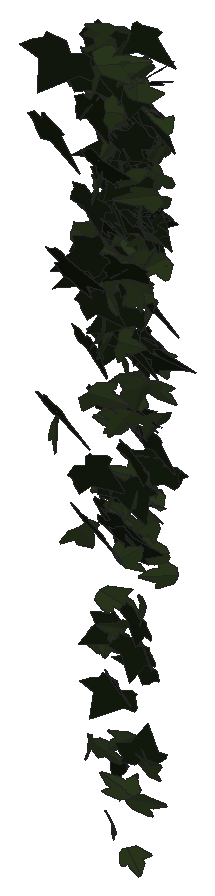
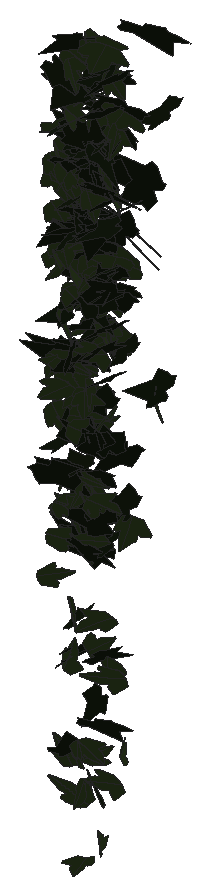
# SketchUp Ruby script. Lengths in millimetres.
U = 1.mm
M = Sketchup.active_model
def pt(a) = Geom::Point3d.new(a.map { |v| v * U })
def face(e, loops, mat)
  f = e.add_face(loops[0].map { |a| pt(a) })
  loops[1..].each { |l| e.add_face(l.map { |a| pt(a) }).erase! }
  f.material = f.back_material = mat if mat
  f
end
# faces: each face lists its corners as indices into pts; further lists are holes
def faces(e, pts, list, mat = nil) = list.each { |f| face(e, (f[0].is_a?(Array) ? f : [f]).map { |l| l.map { |i| pts[i] } }, mat) }
# xy, xz, yz: faces in a plane at the given z, y or x. An outline is a flat list of corners, or four numbers for a rectangle; further outlines are holes
def ring(l) = l.size == 4 ? [[l[0], l[1]], [l[2], l[1]], [l[2], l[3]], [l[0], l[3]]] : l.each_slice(2).to_a
def flat(e, list, mat, &to3) = list.each { |f| face(e, (f[0].is_a?(Array) ? f : [f]).map { |l| ring(l).map { |u, v| to3.(u, v) } }, mat) }
def xy(e, z, list, mat = nil) = flat(e, list, mat) { |x, y| [x, y, z] }
def xz(e, y, list, mat = nil) = flat(e, list, mat) { |x, z| [x, y, z] }
def yz(e, x, list, mat = nil) = flat(e, list, mat) { |y, z| [x, y, z] }
def lines(e, pts, list) = list.each { |a, b| e.add_line(pt(pts[a]), pt(pts[b])) }
# prism: a flat outline (further loops are holes) pulled along v
def prism(e, loops, v, mat = nil)
  f = face(e, loops, mat); d = Geom::Vector3d.new(v.map { |x| x * U })
  f.pushpull(f.normal.samedirection?(d) ? d.length : -d.length)
end
def box(e, o, s, mat = nil) = prism(e, [[o, [o[0] + s[0], o[1], o[2]], [o[0] + s[0], o[1] + s[1], o[2]], [o[0], o[1] + s[1], o[2]]]], [0, 0, s[2]], mat)
def at(x, y, z, deg = 0) = Geom::Transformation.translation(pt([x, y, z])) * Geom::Transformation.rotation(ORIGIN, Z_AXIS, deg.degrees)
def axes(o, x, y, z) = Geom::Transformation.new([*x, 0, *y, 0, *z, 0, *pt(o).to_a, 1])
def part(name) = M.definitions.add(name)
# library, detail: a bought-in or finely detailed component or shape, given as its bounding box
def library(name, o, s) = part(name).tap { |d| box(d.entities, o, s) }
def detail(e, o, s) = box(e.add_group.entities, o, s)
def put(e, d, t, mat = nil) = e.add_instance(d, t).tap { |i| i.material = mat if mat }
def group(e, t, mat = nil) = e.add_group.tap { |g| g.transformation = t; g.material = mat if mat }.entities
root = M.entities
M.materials.add("efeu1").color = [18, 25, 13]
M.materials.add("efeu2").color = [43, 57, 29]
c1 = part("ivyleaf_10")
p = [[0,12.8,-0.8],[-1.5,51.3,-10.9],[-4.9,51,-11.6],[-13.6,26.5,-7.3],[-13.2,15.9,-4.6],[-21.1,19.3,-7.2],
  [-29.5,16.3,-8.3],[-29.2,8.3,-6.2],[-19.7,-9.8,0.5],[-7.6,-13,4],[1,-12.2,5.8],[-0.4,51.1,-11.1],
  [-1.5,51.1,-10.9],[1,-12.4,5.9],[16.9,-12.4,3.5],[35.1,9.1,-5.1],[35,12.9,-6.1],[20.5,16.4,-4.9],
  [15.8,15,-3.8],[15.3,27.6,-7.1],[12.8,31.3,-7.8]]
faces(c1.entities,p,[[0,1,2,3,4,5,6,7,8,9,10],[11,12,0,13,14,15,16,17,18,19,20]],"efeu2")
c2 = part("ivyleaf_9")
p = [[39.1,54.8,31.7],[34.5,51.8,30.2],[-5.3,25.2,17.3],[-17.9,28.3,20.9],[-21.6,21.7,17],[-20.2,4.3,5.3],
  [-22.9,-0.3,2.5],[-17.1,-4,-0.6],[-2,-2.1,-1.2],[-0.7,-15.4,-10.1],[16.6,-22.3,-16.7],[21.1,-15.1,-12.5],
  [32.7,-10.7,-11],[46.1,-1.8,-6.6],[30.8,11.2,3.8]]
faces(c2.entities,p,[[0,1,2,3,4,5,6,7,8,9,10,11,12,13,14]],"efeu1")
put(root,c1,axes([1822.5,943,1481.1],[-0.28005,-0.67314,-0.56509],[0.19497,0.55591,-0.68889],[1.6613,-0.17872,-0.01441]))
put(root,c2,axes([1797.8,841.9,1483.6],[0.91084,-0.90282,-0.01651],[-0.00863,0.01629,-1.02182],[1.71851,0.47859,0.00362]))
put(root,c1,axes([1800.7,982.2,265.7],[-0.64136,0.11442,-0.62069],[1.10096,-0.2254,-0.35563],[-0.48039,-0.66934,0.01365]))
put(root,c2,axes([1805.6,976.5,1322.7],[1.1743,-0.35369,-0.29662],[-0.21622,0.36357,-0.66985],[0.8515,0.58009,0.23897]))
put(root,c2,axes([1832.1,990.5,375.3],[-1.32874,-0.41465,-0.00161],[0.01139,-0.00692,-0.81196],[0.78909,-0.69813,0.00901]))
put(root,c1,axes([1799.8,976.6,463.8],[-0.35998,-0.04208,-0.70449],[1.31314,0.14236,-0.19375],[0.28248,-0.71542,0.00288]))
put(root,c2,axes([1809.5,962.5,1601.2],[0.50907,-0.59476,-0.53681],[-0.20226,0.53459,-0.64527],[1.51135,0.27188,0.09446]))
put(root,c2,axes([1848.5,985.5,1385.8],[-1.38044,0.01635,0.30216],[-0.57495,-0.08465,-0.72058],[0.03342,-0.78117,0.08441]))
put(root,c2,axes([1815.6,968.9,1205],[-0.84219,-0.53442,-0.4027],[0.57762,0.26999,-0.6918],[1.13503,-0.53394,0.05325]))
put(root,c2,axes([1821.2,991.6,1028.3],[-0.43094,-0.70313,0.32913],[-0.17988,-0.31533,-0.73866],[1.46656,-0.24529,0.00611]))
put(root,c2,axes([1808.6,971,1131.2],[0.66553,-0.51406,-0.57933],[-0.15789,0.60713,-0.5888],[1.46559,0.29884,0.19964]))
put(root,c2,axes([1824.8,969.7,1180.9],[0.65454,-0.28914,-0.66596],[-0.91808,0.45971,-0.44871],[1.03266,0.59198,0.02318]))
put(root,c1,axes([1807.4,948.9,1522.4],[1.59505,0.02697,0.36476],[0.69401,0.0092,-0.83852],[-0.05405,0.91398,-0.00232]))
put(root,c1,axes([1830.5,953.2,1584.5],[-0.20352,-0.75394,0.33237],[-0.00832,-0.33464,-0.76049],[1.56813,-0.09963,0.0391]))
put(root,c2,axes([1841.8,974.9,1454.1],[-0.45993,0.76746,0.00714],[-0.00313,0.00697,-0.80461],[-1.46068,-0.24166,-0.00052]))
put(root,c2,axes([1798.8,853.1,959.1],[1.0734,-0.75753,0.18315],[0.21065,-0.14594,-0.94443],[1.46825,0.57475,0.0016]))
put(root,c2,axes([1838.6,980.8,493.7],[-0.77235,-0.44111,0.56041],[-0.71215,-0.41723,-0.59936],[1.15552,-0.55197,0.00519]))
put(root,c2,axes([1807.2,970.2,1194.7],[-0.1034,-0.1559,-0.79226],[0.67159,0.70962,-0.16383],[1.38222,-0.35645,0.02034]))
put(root,c1,axes([1818.5,954.9,1244.4],[1.19737,0.42133,0.11867],[0.16739,0.08188,-0.75695],[-0.81609,0.63497,0.01886]))
put(root,c2,axes([1810.4,979.1,718.9],[0.86688,-0.63563,-0.11104],[-0.12018,0.09135,-0.78198],[1.22216,0.45984,0.00186]))
put(root,c2,axes([1810.2,983.5,901.5],[-0.25854,-0.26803,0.76169],[0.66502,-0.71584,-0.18958],[1.38544,0.29359,0.23314]))
put(root,c1,axes([1818.7,935.2,294.5],[0.06632,-0.01536,0.72305],[0.69663,-0.62395,-0.03089],[1.18711,0.36701,-0.02227]))
put(root,c1,axes([1797.2,939.3,1232.4],[0.25186,-0.01742,0.84861],[1.60609,0.09486,-0.12965],[-0.17334,0.85361,0.03173]))
put(root,c1,axes([1813.9,851.1,925.9],[0.48896,-0.3956,0.84112],[0.97579,-0.66758,-0.47059],[1.47557,0.57256,0.03248]))
put(root,c1,axes([1821.9,972.2,1396],[0.53535,-0.52689,0.55434],[0.53485,-0.47812,-0.59704],[1.35372,0.39727,0.01667]))
put(root,c1,axes([1823,965.1,486.7],[1.22149,-0.19109,0.18532],[0.33707,-0.05457,-0.66965],[0.37822,0.66579,-0.0017]))
put(root,c1,axes([1831,897.6,713.3],[-0.62595,-0.76075,-0.42534],[0.39043,0.37428,-0.82805],[1.6122,-0.38601,0.03539]))
put(root,c2,axes([1840.2,984.2,1072.1],[-0.59749,-0.46681,0.63515],[-0.67582,-0.52662,-0.56255],[1.33933,-0.47397,-0.00051]))
put(root,c2,axes([1807.6,943.5,1536.2],[-0.03607,-0.43085,-0.7109],[1.00024,0.54472,-0.34415],[1.22575,-0.45718,0.25991]))
put(root,c1,axes([1844,978,783.3],[-0.4931,-0.3786,0.71299],[-0.26314,-0.71693,-0.43094],[1.5137,-0.24796,0.15735]))
put(root,c2,axes([1809.1,972.2,1180.6],[0.9158,-0.58167,0.28923],[0.36311,-0.21752,-0.75486],[1.18181,0.51757,0.0078]))
put(root,c2,axes([1825.3,971.6,1359.1],[0.29639,-0.74503,-0.27025],[-0.12894,0.2619,-0.76104],[1.50283,0.16941,-0.01199]))
put(root,c2,axes([1847.8,842.5,1626.5],[-1.75835,-0.45387,-0.15194],[0.26022,0.06627,-1.02935],[0.87296,-0.93395,0.0008]))
put(root,c1,axes([1850.8,975.5,503.2],[-0.38759,-0.1579,-0.65503],[-0.69128,-0.55063,0.24566],[-1.08008,0.40908,0.07783]))
put(root,c2,axes([1859.6,963.4,240.5],[-0.55829,0.20895,-0.70547],[-1.16698,0.35034,0.35873],[0.77395,0.67897,0.032]))
put(root,c1,axes([1836.3,973.6,1124.6],[0.01605,-0.18199,0.7631],[0.40521,-0.73397,-0.1774],[1.43703,0.209,0.0415]))
put(root,c2,axes([1820.6,923.5,1052.3],[0.45536,-0.74582,0.36603],[0.15434,-0.35812,-0.78272],[1.57363,0.25094,-0.02915]))
put(root,c1,axes([1842,963.1,922.1],[-0.25016,0.57468,0.54752],[0.1665,-0.5411,0.58895],[1.50145,0.15575,0.02591]))
put(root,c2,axes([1830.2,979.5,1225],[-0.22156,-0.7799,0.28254],[0.08433,-0.29074,-0.7843],[1.57645,-0.09406,0.08166]))
put(root,c2,axes([1828.8,924.6,1321.6],[-0.02349,-0.81617,0.10867],[0.0394,-0.10895,-0.81596],[1.56655,-0.0095,0.02215]))
put(root,c1,axes([1828.9,977.7,131.6],[-0.35685,0.08828,0.63772],[0.83068,-0.47084,0.19351],[0.90071,0.46921,0.07419]))
put(root,c1,axes([1860.2,933.7,1488.3],[-1.3551,0.11709,0.42797],[-0.81604,0.02654,-0.72061],[-0.21718,-0.83031,0.03732]))
put(root,c1,axes([1847.5,954.4,1412],[0.21003,-0.84178,-0.35734],[-0.06931,0.3556,-0.84893],[1.73907,0.11584,0.00932]))
put(root,c2,axes([1832.4,974.7,1530.9],[-0.19851,-0.80782,-0.10846],[0.03186,0.1072,-0.81452],[1.55092,-0.1056,0.00285]))
put(root,c2,axes([1831.1,946.9,1213.4],[0.94597,-0.38709,-0.5058],[-0.45391,0.4818,-0.60309],[1.124,0.52034,0.18214]))
put(root,c2,axes([1824.1,932,1489.5],[-0.53964,-0.16781,-0.80142],[1.55793,-0.03867,-0.28152],[0.0357,-0.84922,0.17118]))
put(root,c1,axes([1839.2,935.7,1353.4],[0.56258,-0.62662,0.51847],[0.42502,-0.46791,-0.69284],[1.48839,0.37047,0.00187]))
put(root,c2,axes([1837.2,968.8,1440.7],[-0.30047,-0.49117,0.63866],[0.01681,-0.65182,-0.49911],[1.53329,-0.08911,0.13063]))
put(root,c2,axes([1820.7,930.9,1281.7],[0.3083,-0.37225,0.7742],[0.69931,-0.68211,-0.40485],[1.47782,0.40044,0.03006]))
put(root,c2,axes([1858.6,974.8,1162.7],[-0.58438,0.64426,-0.3801],[0.3307,-0.3382,-0.71362],[-1.38471,-0.35266,-0.01002]))
put(root,c1,axes([1853.3,980.5,1363.8],[-0.25887,-0.80427,-0.03819],[-0.00137,0.03885,-0.81566],[1.53242,-0.13583,-0.00718]))
put(root,c1,axes([1831.7,967.6,560.8],[0.56824,0.42412,0.62452],[0.58902,0.54379,-0.51725],[-1.31047,0.42832,0.03831]))
put(root,c2,axes([1846,962.8,407.6],[1.14893,-0.26922,-0.47629],[-0.83014,0.19133,-0.66099],[0.62859,0.74477,-0.00236]))
put(root,c2,axes([1824.5,982.3,893.2],[-0.00837,0.01,0.7808],[1.31996,-0.35873,0.0085],[0.68288,0.69353,-0.00686]))
put(root,c1,axes([1855.5,959.5,1498.5],[-0.26483,-0.74986,0.33585],[0.07633,-0.34643,-0.75686],[1.56188,-0.11022,0.09394]))
put(root,c1,axes([1829.6,977.8,715.6],[0.57678,0.07748,0.6264],[1.12171,0.21391,-0.31161],[-0.42985,0.66217,0.02737]))
put(root,c1,axes([1835.1,980.9,1072.2],[-0.85041,0.0973,-0.60337],[1.05014,-0.25716,-0.4501],[-0.50015,-0.70539,0.08087]))
put(root,c1,axes([1870.6,938.8,1630.9],[-1.16692,-0.45216,0.3727],[-0.50315,-0.26795,-0.76],[0.99525,-0.66562,0.05277]))
put(root,c2,axes([1841.7,910.3,1148.3],[0.52178,-0.5404,-0.6401],[-0.27287,0.6333,-0.59607],[1.57081,0.28952,0.10908]))
put(root,c1,axes([1861.3,912.1,1087.4],[0.15621,-0.72855,-0.48451],[-0.0897,0.48225,-0.73314],[1.66279,0.09446,0.00597]))
put(root,c1,axes([1854.2,943.5,1625.9],[-1.2911,-0.4395,-0.24822],[0.4042,0.12868,-0.80828],[0.87146,-0.71082,0.00715]))
put(root,c2,axes([1851.9,973.9,1428.4],[-0.46239,0.17122,-0.76702],[1.07645,-0.51932,-0.29508],[-1.03848,-0.61454,0.03566]))
put(root,c2,axes([1857.1,986.5,699.8],[-1.28707,-0.11085,-0.41353],[0.77393,0.07549,-0.68525],[0.25485,-0.78908,-0.00747]))
put(root,c2,axes([1846.3,941.8,1575.7],[-0.48594,-0.75949,-0.34593],[0.29742,0.31185,-0.80001],[1.56024,-0.29599,0.04476]))
put(root,c1,axes([1861.8,972.6,998.7],[0.6302,-0.44636,-0.5607],[-0.13184,0.59483,-0.51444],[1.35758,0.26497,0.21032]))
put(root,c2,axes([1828.6,955,1235.7],[0.26393,-0.13524,-0.79554],[1.19089,0.52773,0.01937],[0.96977,-0.61125,0.19273]))
put(root,c1,axes([1852.4,963.7,1211.1],[-0.41267,-0.52961,-0.55132],[0.5706,0.46825,-0.56772],[1.33841,-0.36292,0.07205]))
put(root,c2,axes([1850.6,984.9,1165.4],[-0.16514,-0.62892,0.45455],[-0.07873,-0.45299,-0.63465],[1.47476,-0.09461,0.01702]))
put(root,c2,axes([1828,972.4,748.1],[0.84176,-0.04822,0.63431],[1.19663,-0.08427,-0.44482],[0.184,0.76867,-0.00898]))
put(root,c1,axes([1873,972.9,309.3],[-0.6641,-0.40693,0.41414],[-0.49373,-0.32299,-0.53595],[0.98857,-0.43468,0.01053]))
put(root,c1,axes([1859.5,942.9,1426.2],[0.89336,-0.69261,0.04582],[0.04127,-0.04066,-0.83667],[1.32041,0.46988,-0.00485]))
put(root,c1,axes([1864.6,952.8,1433.1],[-0.27859,-0.67822,0.52747],[0.04806,-0.53823,-0.68505],[1.6345,-0.09977,0.11005]))
put(root,c1,axes([1856.5,971.8,908.1],[0.10651,-0.34727,0.61371],[0.39166,-0.5808,-0.34741],[1.28362,0.20603,0.05508]))
put(root,c1,axes([1857.6,913.9,1573.6],[0.19868,-0.73708,0.41387],[0.37639,-0.38414,-0.73402],[1.56417,0.18606,0.12406]))
put(root,c1,axes([1865.6,971.4,1232],[-0.32409,-0.73889,-0.09967],[0.01445,0.10052,-0.75811],[1.41892,-0.16979,-0.01505]))
put(root,c2,axes([1847.2,969.5,1297.5],[0.15955,-0.67692,-0.36171],[0.09908,0.36804,-0.6767],[1.45734,0.04909,0.0856]))
put(root,c2,axes([1852.4,886,842.6],[0.24473,-0.32835,-0.91099],[-0.41175,0.88602,-0.34989],[1.79639,0.24781,0.04391]))
put(root,c2,axes([1864.7,952.5,1297.8],[1.33185,0.05372,-0.52183],[-0.98889,-0.04871,-0.70182],[-0.13736,0.87158,-0.00706]))
put(root,c1,axes([1872,949.5,902.5],[0.07884,0.41072,0.69902],[-0.24377,-0.68783,0.41173],[1.52365,-0.1313,0.0297]))
put(root,c1,axes([1865.9,977.1,976.2],[-0.60914,-0.61883,-0.10988],[0.14236,0.08493,-0.69617],[1.18768,-0.32757,0.02709]))
put(root,c2,axes([1853.7,991.1,1448.1],[-0.22963,-0.66474,0.43452],[0.08103,-0.44429,-0.66786],[1.50926,-0.07728,0.10197]))
put(root,c1,axes([1881.2,979.3,938.1],[0.23799,0.11534,-0.73489],[-1.08954,-0.46092,-0.16976],[-0.90403,0.58587,0.01113]))
put(root,c2,axes([1833.9,963.9,1213.6],[1.26474,-0.16089,0.42007],[0.78731,-0.07577,-0.68343],[0.33628,0.78251,0.02019]))
put(root,c1,axes([1839.5,938,1153.6],[0.84514,-0.23107,0.71757],[1.25425,-0.28539,-0.49973],[0.69666,0.79413,0.0292]))
put(root,c1,axes([1867.2,918.8,1069.4],[0.42465,-0.83713,0.09685],[0.02521,-0.09669,-0.86627],[1.60366,0.22319,-0.01203]))
put(root,c2,axes([1847.3,975.9,1479.8],[0.58263,-0.76598,-0.00762],[-0.00221,0.00774,-0.82489],[1.45789,0.30613,0.0018]))
put(root,c1,axes([1874.1,991.7,919.8],[-0.30434,-0.41095,0.66463],[-0.16009,-0.66541,-0.43167],[1.47854,-0.15663,0.09007]))
put(root,c2,axes([1834.6,962.4,706.8],[0.53386,0.03211,-0.76052],[1.41685,0.15749,0.28123],[0.30217,-0.79516,0.02499]))
put(root,c2,axes([1841.4,927.8,1377],[0.11329,-0.17813,0.8059],[0.85649,-0.67031,-0.1814],[1.31676,0.45133,0.04866]))
put(root,c1,axes([1887.2,925.4,1195],[0.68071,-0.04272,0.68291],[-1.24009,0.21396,0.35464],[-0.39753,-0.74061,0.06307]))
put(root,c1,axes([1881,954.1,690.9],[-0.91257,0.27866,0.43713],[-0.71416,0.22425,-0.55457],[-0.68071,-0.60885,-0.00419]))
put(root,c2,axes([1847.9,978.3,923.8],[-0.3637,-0.02871,-0.79209],[1.50732,-0.03908,-0.18966],[-0.05954,-0.81388,0.03705]))
put(root,c2,axes([1852.5,963.8,1580.5],[-0.23105,-0.57329,0.59413],[0.41054,-0.60168,-0.5365],[1.51674,0.07553,0.23572]))
put(root,c2,axes([1840.5,896.9,737.6],[0.81306,-0.74552,0.44349],[0.40556,-0.38901,-0.85921],[1.60035,0.47735,-0.00757]))
put(root,c2,axes([1862.5,986.2,1420.8],[-0.21939,-0.45927,0.64404],[-0.1398,-0.64181,-0.47083],[1.49896,-0.12708,0.05035]))
put(root,c2,axes([1875.9,968.2,1109.4],[-0.85346,-0.60059,0.32634],[-0.35252,-0.26892,-0.74945],[1.25221,-0.48505,0.01144]))
put(root,c1,axes([1866.9,945,783.1],[0.41901,-0.65504,0.51825],[0.32363,-0.48957,-0.69103],[1.55637,0.27815,0.00417]))
put(root,c2,axes([1894,859.4,1263.4],[-1.66077,0.45668,-0.06416],[0.10435,-0.03359,-0.98488],[-0.87146,-0.87433,0.00433]))
put(root,c1,axes([1870.8,934.3,1208.6],[-1.30302,-0.55594,-0.24115],[0.35021,0.15593,-0.88192],[1.09886,-0.70893,-0.00488]))
put(root,c2,axes([1893.9,856,1238],[-1.58067,0.51141,-0.15074],[0.24046,-0.0823,-0.97535],[-0.98581,-0.84008,0.00379]))
put(root,c1,axes([1872.5,971.2,782.2],[0.50481,-0.63065,0.18301],[0.17767,-0.15916,-0.68375],[1.23707,0.28021,0.02352]))
put(root,c1,axes([1872.9,969.4,794.7],[-0.1828,-0.46352,-0.58755],[0.36361,0.55755,-0.47108],[1.3771,-0.20874,0.04639]))
put(root,c1,axes([1879.6,986.8,1396.9],[-0.5042,-0.62399,0.42829],[0.16651,-0.47597,-0.63936],[1.43075,-0.1645,0.22534]))
put(root,c2,axes([1867.4,954.5,1300.8],[-0.53794,-0.70283,-0.44801],[0.28928,0.42167,-0.7574],[1.55967,-0.32062,-0.01404]))
put(root,c1,axes([1870.6,975.1,92.7],[0.50928,0.63699,0.15355],[0.11537,0.14108,-0.69091],[-1.2417,0.27437,-0.00122]))
put(root,c1,axes([1879.4,986.9,1218.2],[0.21671,-0.65451,0.3887],[0.1086,-0.38458,-0.66429],[1.44469,0.12709,-0.00837]))
put(root,c1,axes([1878.4,964.3,226.1],[-0.15884,-0.55043,-0.56858],[0.23112,0.55605,-0.55613],[1.48829,-0.1451,0.02568]))
put(root,c1,axes([1904.6,958.3,808.8],[-0.17355,0.13167,0.69466],[-1.26071,-0.26077,-0.03753],[0.47041,-0.65028,0.1557]))
put(root,c1,axes([1907,960.2,1154.6],[0.24741,0.01854,-0.7798],[-1.4631,0.13692,-0.1249],[0.25139,0.77862,0.04053]))
put(root,c2,axes([1869.4,989.6,1164.7],[0.0492,-0.73587,0.19095],[0.00312,-0.191,-0.73631],[1.44689,0.02544,-0.00491]))
put(root,c2,axes([1854.5,988.5,1476.3],[0.13145,-0.43212,0.67428],[1.00864,-0.48274,-0.36366],[1.14273,0.4758,0.24342]))
put(root,c2,axes([1871,985.5,1412.3],[-0.87734,-0.32625,-0.55242],[0.85773,0.31946,-0.56475],[0.86902,-0.64468,-0.0003]))
put(root,c1,axes([1872.6,948.6,1383.8],[-0.08659,0.1218,-0.82294],[0.29384,-0.80861,-0.12822],[-1.55577,-0.1595,0.02159]))
put(root,c1,axes([1885.5,982.8,974.1],[0.33674,0.46418,-0.50116],[-0.37947,-0.46006,-0.49651],[-1.24347,0.2661,0.0158]))
put(root,c2,axes([1889.3,986.7,1315.7],[-0.88968,-0.46715,0.42333],[-0.21195,-0.45753,-0.62787],[1.18096,-0.43405,0.20623]))
put(root,c2,axes([1869.9,982.8,1363.5],[0.74048,-0.64319,-0.29751],[-0.20409,0.28206,-0.75002],[1.3332,0.40042,0.05043]))
put(root,c2,axes([1864.8,963.7,771.7],[1.35884,-0.31497,0.00674],[0.01787,0.0046,-0.78032],[0.59933,0.71399,0.008]))
put(root,c2,axes([1889,991,1426.6],[-1.1084,-0.55228,-0.01289],[0.11874,-0.04714,-0.7989],[1.04466,-0.58062,0.07713]))
put(root,c2,axes([1880.6,971.9,1457.1],[-1.17678,-0.20887,-0.52588],[0.92384,0.20449,-0.65196],[0.55339,-0.78553,-0.02989]))
put(root,c2,axes([1877.2,981.7,1046.5],[-0.06734,-0.57911,0.57544],[-0.10267,-0.57307,-0.58004],[1.55038,-0.06311,-0.01342]))
put(root,c2,axes([1880.3,951.9,1324.5],[-0.38321,-0.86009,0.05611],[-0.01686,-0.05555,-0.88334],[1.64032,-0.20151,0.00403]))
put(root,c1,axes([1880.5,909.2,1501.2],[0.23015,-0.37086,-0.76013],[0.60574,0.73137,-0.30619],[1.49135,-0.23983,0.24167]))
put(root,c2,axes([1903.6,943.1,1304.8],[-0.5287,0.34432,-0.75773],[-1.06723,0.51287,0.43864],[1.17054,0.62313,0.05767]))
put(root,c2,axes([1873.6,951.5,1333.4],[0.60257,-0.66111,-0.34983],[-0.13909,0.35072,-0.72893],[1.41671,0.31562,0.07723]))
put(root,c2,axes([1899.8,952.3,1370.8],[-1.28202,-0.47936,0.12079],[-0.17346,-0.08023,-0.82667],[0.92471,-0.67964,0.01239]))
put(root,c2,axes([1876.6,971.1,1060.4],[-0.94977,-0.31405,-0.64784],[1.06686,0.32513,-0.58942],[0.8598,-0.75035,0.01574]))
put(root,c2,axes([1885.5,969.6,1324.5],[-0.7429,-0.6629,-0.13299],[0.22461,0.08441,-0.7671],[1.26701,-0.40365,0.05801]))
put(root,c1,axes([1899.2,971.5,1157.7],[-0.30352,-0.64811,0.46925],[-0.1373,-0.46488,-0.66659],[1.51664,-0.17179,0.03357]))
put(root,c1,axes([1913.1,953,1264.4],[-0.85321,-0.37107,0.57593],[-0.86084,-0.35666,-0.58187],[0.97937,-0.63676,-0.00971]))
put(root,c1,axes([1895.9,928.5,1626.4],[0.27303,-0.84014,-0.04863],[-0.02499,0.04709,-0.85228],[1.60143,0.14397,-0.00501]))
put(root,c2,axes([1906.3,906.7,1228.7],[0.76459,0.40152,-0.67045],[-0.87842,-0.48643,-0.56788],[-1.20022,0.61179,-0.01149]))
put(root,c1,axes([1872.2,984.3,291.4],[0.15248,-0.0853,0.72007],[1.13421,-0.40495,-0.11428],[0.78615,0.60078,0.02521]))
put(root,c1,axes([1896.7,982.7,461.4],[-1.13772,0.61678,0.09343],[0.11243,-0.07284,0.8589],[1.1819,0.60065,0.00823]))
put(root,c2,axes([1865.3,928.1,937.3],[0.56261,-0.55547,0.55692],[0.68669,-0.43291,-0.6233],[1.33022,0.45841,0.08621]))
put(root,c2,axes([1884.8,995,1057.9],[-0.03263,0.05335,-0.77052],[1.02523,-0.55149,-0.05017],[-1.05343,-0.53838,-0.02497]))
put(root,c2,axes([1884.9,959.8,1525],[-0.40546,-0.72041,0.36821],[0.10203,-0.39249,-0.7369],[1.5364,-0.16406,0.14611]))
put(root,c2,axes([1921.6,973.5,1279.1],[-1.21383,-0.06359,0.51912],[-0.97235,-0.09932,-0.63985],[0.21286,-0.81633,0.03741]))
put(root,c2,axes([1873.1,977.1,1465.5],[0.40928,-0.71302,0.35637],[0.27691,-0.3278,-0.74365],[1.49158,0.2565,0.04027]))
put(root,c1,axes([1895.8,975.3,1507],[0.10873,-0.63947,0.49199],[0.0998,-0.48924,-0.64198],[1.53231,0.07724,0.0069]))
put(root,c2,axes([1866.5,981.9,912.7],[1.19256,-0.09736,-0.53106],[0.98932,-0.11112,0.63371],[-0.27776,-0.81383,-0.023]))
put(root,c2,axes([1875.7,949.5,1066.6],[1.00391,-0.70618,-0.17102],[-0.15354,0.15311,-0.88103],[1.3743,0.53296,0.0265]))
put(root,c2,axes([1890.9,963.2,486.9],[-0.43314,-0.74793,0.15072],[-0.09074,-0.14304,-0.78178],[1.44925,-0.23249,-0.0039]))
put(root,c1,axes([1917.9,985.5,1037.5],[-0.56384,-0.13598,0.66689],[-0.97512,-0.43421,-0.31615],[0.85266,-0.58649,0.07944]))
put(root,c1,axes([1903.5,985.2,1404.5],[-0.29781,-0.72443,0.28072],[-0.12226,-0.27332,-0.74112],[1.47357,-0.16909,-0.00476]))
put(root,c1,axes([1901.1,978.7,1382.8],[1.41242,-0.09213,-0.2567],[-0.41514,0.24621,-0.71899],[0.31158,0.74567,0.20568]))
put(root,c1,axes([1906.5,988.4,767.8],[0.54139,0.31832,-0.64202],[-0.77354,-0.49723,-0.42662],[-1.12325,0.49585,-0.01565]))
put(root,c1,axes([1903.5,991,766.4],[-0.37028,-0.54533,0.44438],[-0.07635,-0.45172,-0.57189],[1.33665,-0.17687,0.09044]))
put(root,c1,axes([1907.6,916.6,247.5],[0.56397,0.50117,0.46093],[-0.43889,-0.39911,0.58221],[1.21931,-0.37547,-0.00363]))
put(root,c1,axes([1908.4,918.4,943.1],[-0.74445,-0.67084,0.38941],[-0.22119,-0.38051,-0.77226],[1.4596,-0.39982,0.08158]))
put(root,c2,axes([1882.7,966.6,1499.5],[0.30353,-0.78413,-0.19331],[0.02554,0.19959,-0.79853],[1.53683,0.15155,0.05145]))
put(root,c1,axes([1904.5,964.6,565.1],[0.44321,-0.544,-0.47698],[-0.19409,0.4714,-0.58742],[1.36321,0.24398,0.07144]))
put(root,c2,axes([1883.6,972.4,834],[-0.10043,-0.63435,0.54605],[0.25756,-0.5464,-0.62168],[1.57202,0.049,0.13674]))
put(root,c2,axes([1890.9,967.3,538.7],[-0.102,-0.62249,0.51238],[-0.07901,-0.5107,-0.62479],[1.53241,-0.06777,0.00189]))
put(root,c2,axes([1897.7,924,1202.9],[0.5849,0.52797,0.47533],[0.37686,0.43372,-0.60977],[-1.29848,0.3637,0.03714]))
put(root,c2,axes([1903.3,965.2,284.1],[-0.9833,-0.2467,0.52778],[0.90892,0.22467,0.57253],[-0.63504,0.70357,0.00224]))
put(root,c2,axes([1910.1,972.1,457.2],[0.09153,-0.68008,-0.3633],[0.10886,-0.35985,0.6812],[-1.46339,-0.06931,0.02795]))
put(root,c2,axes([1894.3,945.3,1292.7],[-0.3798,-0.3993,0.67243],[0.097,-0.69914,-0.40004],[1.48524,-0.05645,0.19808]))
put(root,c2,axes([1892.7,953.9,1427.2],[-0.48518,-0.59695,0.62262],[0.22651,-0.66737,-0.59113],[1.62592,-0.08516,0.26815]))
put(root,c1,axes([1908.2,961.1,1585.4],[-0.12232,-0.83592,-0.05428],[0.01236,0.05394,-0.83838],[1.59423,-0.06455,0.00233]))
put(root,c1,axes([1909.7,984,1257.4],[-0.66736,-0.6925,0.04126],[-0.02586,-0.03937,-0.7762],[1.32005,-0.35087,0.00566]))
put(root,c2,axes([1877.9,956.2,677.5],[0.15386,-0.10708,0.80382],[0.94433,-0.6324,-0.13415],[1.22071,0.50271,0.00246]))
put(root,c1,axes([1919.1,950,994.3],[-1.00101,-0.47765,0.32754],[-0.47041,-0.21501,-0.71046],[0.99685,-0.58111,-0.00636]))
put(root,c1,axes([1906,988.5,1113],[0.65491,-0.78039,0.13756],[0.07173,-0.13369,-0.85267],[1.50643,0.34563,-0.0192]))
put(root,c2,axes([1936.2,915.7,1450],[-0.78376,0.50465,0.61171],[-0.75693,0.46488,-0.65127],[-1.30572,-0.57242,0.01037]))
put(root,c1,axes([1900.8,937.6,785.5],[1.00899,-0.61555,0.24235],[0.29143,-0.18795,-0.81236],[1.22485,0.55179,-0.00635]))
put(root,c2,axes([1891.7,988,1257.1],[0.33166,-0.73716,-0.12165],[-0.00012,0.1249,-0.75695],[1.42193,0.17195,0.02831]))
put(root,c2,axes([1893.7,933.4,806.7],[-0.69808,-0.49197,-0.58723],[0.67652,0.46744,-0.61364],[1.29155,-0.51076,0.00403]))
put(root,c1,axes([1883.2,964.5,201.4],[-0.69563,-0.1091,0.69788],[1.3165,0.10379,0.37851],[-0.27215,0.78093,0.04719]))
put(root,c1,axes([1896.6,938.2,1370.8],[-0.6245,-0.39133,-0.71261],[0.84081,0.55927,-0.51055],[1.2989,-0.55018,-0.01212]))
put(root,c2,axes([1893.6,991.6,1269.9],[0.19893,-0.68012,0.38885],[0.05178,-0.38891,-0.68753],[1.49013,0.10431,-0.02802]))
put(root,c2,axes([1928.8,986.6,825.1],[0.20647,0.17324,-0.78605],[-0.71666,-0.69008,-0.20406],[-1.35393,0.39169,-0.01186]))
put(root,c2,axes([1898.1,983.1,1263.4],[-0.29866,-0.61523,0.48098],[0.24601,-0.50429,-0.60287],[1.46576,-0.04072,0.19919]))
put(root,c2,axes([1906.1,951.4,1544.7],[1.03381,0.54528,0.27712],[0.09498,0.32988,-0.74691],[-1.16023,0.51287,0.18578]))
put(root,c1,axes([1881.4,902.5,1593.4],[0.74144,-0.03538,-0.83311],[1.52528,0.26982,0.36331],[0.43826,-0.87922,0.14501]))
put(root,c1,axes([1899.6,957.7,1302],[-0.08474,0.21512,-0.78538],[0.4532,-0.74873,-0.21858],[-1.48205,-0.24126,-0.02193]))
put(root,c2,axes([1909.2,959.4,1285.2],[-0.06677,0.18184,-0.90896],[-0.53395,0.86486,0.18385],[1.68146,0.28186,0.02229]))
put(root,c1,axes([1914.4,988.1,1242.4],[0.24277,-0.69093,0.30369],[0.07561,-0.30143,-0.70246],[1.4344,0.13283,-0.01437]))
put(root,c2,axes([1898,985.9,1288.3],[0.07665,-0.7129,-0.31599],[0.15087,0.31852,-0.70849],[1.47642,0.00446,0.0888]))
put(root,c1,axes([1916,939.1,1535],[1.56713,-0.1898,0.24829],[-0.43032,0.12125,0.84253],[-0.41061,-0.85145,0.06463]))
put(root,c1,axes([1897,924.7,673],[1.08837,-0.21838,-0.37785],[0.6653,-0.14367,0.61209],[-0.49726,-0.67019,-0.00809]))
put(root,c1,axes([1906.8,909,1082.4],[0.03127,-0.49016,-0.7341],[0.66784,0.67734,-0.44441],[1.5415,-0.28351,0.20743]))
put(root,c1,axes([1926,968.8,1370.6],[-1.23533,-0.41453,0.17804],[-0.24245,-0.13085,-0.76908],[0.82369,-0.66021,0.04064]))
put(root,c1,axes([1921.4,955.2,1262.9],[-0.30151,-0.79178,0.00963],[-0.00438,-0.00936,-0.80747],[1.50702,-0.15844,-0.00042]))
put(root,c1,axes([1938,963.2,679.4],[-0.24328,-0.02624,0.7514],[-0.94421,-0.56976,-0.10429],[1.0752,-0.50628,0.07843]))
put(root,c2,axes([1897.4,948.2,1635.1],[0.17718,-0.46332,-0.70698],[0.31557,0.70745,-0.44179],[1.57747,-0.08948,0.16779]))
put(root,c2,axes([1896.8,979.8,1130.6],[1.02868,-0.61004,-0.03095],[-0.03715,0.02405,-0.81504],[1.16194,0.54085,0.00134]))
put(root,c2,axes([1930.9,978.7,831.2],[-1.51578,-0.34036,0.05383],[-0.09124,-0.02479,-0.86611],[0.64945,-0.79787,0.00395]))
put(root,c1,axes([1901,949.3,1233.3],[0.72627,0.27253,-0.68362],[0.88687,0.50654,0.46206],[1.08409,-0.59697,0.07998]))
put(root,c1,axes([1918.5,960.8,811.3],[-0.67575,0.58791,0.17196],[-0.15864,0.15054,-0.68678],[-1.15495,-0.36466,-0.00628]))
put(root,c1,axes([1924.4,982.3,1319.4],[-0.52879,-0.67667,0.26113],[-0.08239,-0.26367,-0.72929],[1.37794,-0.27544,0.05661]))
put(root,c1,axes([1929.8,932.8,1590.6],[-0.32015,-0.65469,0.56834],[-0.31419,-0.54416,-0.6757],[1.61982,-0.23494,-0.01873]))
put(root,c1,axes([1939.3,940.5,1350.9],[0.41627,0.23197,-0.72314],[-1.25992,-0.31052,-0.29984],[-0.70825,0.68873,0.10837]))
put(root,c1,axes([1912.8,971.8,1216.3],[-0.04537,-0.46359,-0.65844],[0.52881,0.61354,-0.44204],[1.43847,-0.24017,0.14173]))
put(root,c1,axes([1905,967.6,270.1],[-1.03456,0.03892,0.52665],[0.9632,-0.17745,0.53549],[0.28702,0.73578,0.10129]))
put(root,c1,axes([1908.1,835.4,1020],[-0.67599,-0.42275,-0.82011],[1.01075,0.62493,-0.55215],[1.43594,-0.6389,0.00258]))
put(root,c1,axes([1932.6,948.8,742],[1.01866,-0.52888,-0.44565],[-0.53021,0.3509,-0.75103],[1.20475,0.60162,0.04628]))
put(root,c1,axes([1927.2,985.9,1411.8],[-0.33921,-0.78364,0.13694],[0.00035,-0.14038,-0.80306],[1.51402,-0.17554,0.03087]))
put(root,c1,axes([1927.1,920.2,1176.2],[0.9653,-0.51492,-0.27783],[-0.23669,0.2644,-0.71708],[1.08809,0.51432,0.09049]))
put(root,c2,axes([1905.2,975.8,883.1],[0.71375,-0.69769,-0.07409],[-0.06919,0.06457,-0.7921],[1.33352,0.37678,-0.00145]))
put(root,c1,axes([1927.8,923.2,992.2],[-0.48242,-0.82349,-0.10141],[0.06256,0.09598,-0.86161],[1.57786,-0.25558,0.00316]))
put(root,c1,axes([1933.7,996.3,621.4],[-0.07137,0.11701,0.77345],[-0.31318,-0.75819,0.10673],[1.45547,-0.15741,0.06089]))
put(root,c1,axes([1931.6,969.4,1460.6],[0.69121,0.69126,0.2309],[-0.31185,-0.17393,0.77843],[1.35154,-0.39365,0.06152]))
put(root,c2,axes([1892.6,964.5,1028.7],[0.48789,-0.15699,0.75804],[1.24207,-0.38565,-0.30057],[0.79241,0.70115,0.0044]))
put(root,c1,axes([1932.5,970.6,925.7],[-0.42999,-0.81988,0.2014],[-0.11375,-0.19243,-0.85042],[1.60276,-0.23362,-0.00633]))
put(root,c2,axes([1885.7,777.9,1279.4],[1.38786,-0.18794,-0.82004],[1.57563,-0.03275,0.74371],[-0.28485,-1.09689,0.1183]))
put(root,c1,axes([1917.8,976.8,1028.7],[0.5028,0.63454,0.30145],[0.12415,0.29851,-0.68552],[-1.33123,0.2675,0.04992]))
put(root,c1,axes([1914.5,973.2,976.7],[-1.04258,-0.12381,-0.44],[0.80542,0.12217,-0.56125],[0.32876,-0.69193,-0.02037]))
put(root,c2,axes([1909.2,975,1483.1],[0.5726,-0.772,-0.06699],[-0.03728,0.06427,-0.82854],[1.47432,0.30146,0.00507]))
put(root,c2,axes([1940.7,964,1575.8],[-0.63293,0.6112,-0.43787],[0.23559,-0.42775,-0.69109],[-1.41142,-0.34548,0.081]))
put(root,c2,axes([1895.5,982.7,1037.8],[0.7959,-0.27883,0.62322],[0.9675,-0.36071,-0.50249],[0.86743,0.65816,-0.01137]))
put(root,c1,axes([1931.1,949.3,1237.8],[-0.14255,-0.68433,0.41502],[0.08401,-0.41973,-0.68413],[1.52089,-0.04096,0.07669]))
put(root,c1,axes([1941.6,962.8,1220.7],[0.45456,0.37614,-0.75357],[-0.96473,-0.56134,-0.44084],[-1.28011,0.55661,0.06465]))
put(root,c1,axes([1930.3,967.7,1425.4],[0.35221,-0.79542,0.11417],[0.07165,-0.10845,-0.81658],[1.52768,0.18848,0.01198]))
